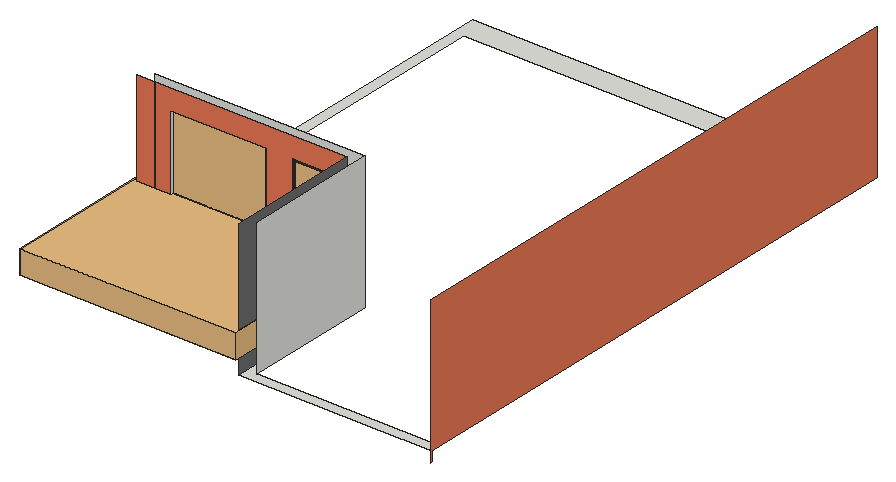
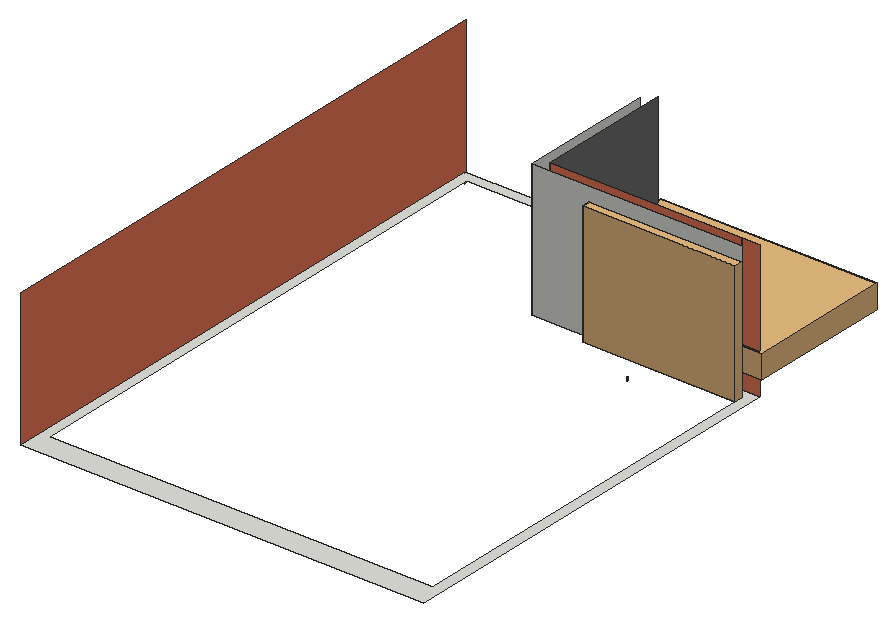
# SketchUp Ruby script. Lengths in inches.
U = 1.inch
M = Sketchup.active_model
def pt(a) = Geom::Point3d.new(a.map { |v| v * U })
def face(e, loops, mat)
  f = e.add_face(loops[0].map { |a| pt(a) })
  loops[1..].each { |l| e.add_face(l.map { |a| pt(a) }).erase! }
  f.material = f.back_material = mat if mat
  f
end
# faces: each face lists its corners as indices into pts; further lists are holes
def faces(e, pts, list, mat = nil) = list.each { |f| face(e, (f[0].is_a?(Array) ? f : [f]).map { |l| l.map { |i| pts[i] } }, mat) }
# xy, xz, yz: faces in a plane at the given z, y or x. An outline is a flat list of corners, or four numbers for a rectangle; further outlines are holes
def ring(l) = l.size == 4 ? [[l[0], l[1]], [l[2], l[1]], [l[2], l[3]], [l[0], l[3]]] : l.each_slice(2).to_a
def flat(e, list, mat, &to3) = list.each { |f| face(e, (f[0].is_a?(Array) ? f : [f]).map { |l| ring(l).map { |u, v| to3.(u, v) } }, mat) }
def xy(e, z, list, mat = nil) = flat(e, list, mat) { |x, y| [x, y, z] }
def xz(e, y, list, mat = nil) = flat(e, list, mat) { |x, z| [x, y, z] }
def yz(e, x, list, mat = nil) = flat(e, list, mat) { |y, z| [x, y, z] }
def lines(e, pts, list) = list.each { |a, b| e.add_line(pt(pts[a]), pt(pts[b])) }
# prism: a flat outline (further loops are holes) pulled along v
def prism(e, loops, v, mat = nil)
  f = face(e, loops, mat); d = Geom::Vector3d.new(v.map { |x| x * U })
  f.pushpull(f.normal.samedirection?(d) ? d.length : -d.length)
end
def box(e, o, s, mat = nil) = prism(e, [[o, [o[0] + s[0], o[1], o[2]], [o[0] + s[0], o[1] + s[1], o[2]], [o[0], o[1] + s[1], o[2]]]], [0, 0, s[2]], mat)
def at(x, y, z, deg = 0) = Geom::Transformation.translation(pt([x, y, z])) * Geom::Transformation.rotation(ORIGIN, Z_AXIS, deg.degrees)
def axes(o, x, y, z) = Geom::Transformation.new([*x, 0, *y, 0, *z, 0, *pt(o).to_a, 1])
def part(name) = M.definitions.add(name)
# library, detail: a bought-in or finely detailed component or shape, given as its bounding box
def library(name, o, s) = part(name).tap { |d| box(d.entities, o, s) }
def detail(e, o, s) = box(e.add_group.entities, o, s)
def put(e, d, t, mat = nil) = e.add_instance(d, t).tap { |i| i.material = mat if mat }
def group(e, t, mat = nil) = e.add_group.tap { |g| g.transformation = t; g.material = mat if mat }.entities
root = M.entities
M.materials.add("1122 AP 7994 PEACH ROSE").color = [254, 227, 201]
M.materials.add("[Formica Beige]").color = [235, 120, 86]
M.materials.add("[Metal Rusted]").color = [135, 86, 63]
M.materials.add("[Stone Flagstone Ashlar]").color = [109, 109, 109]
M.materials.add("[Translucent Glass Blue]1").color = [190, 201, 222]
M.materials["[Translucent Glass Blue]1"].alpha = 0.5
M.materials.add("[Wood Veneer 01]").color = [96, 60, 36]
c1 = library("Group\#47",[0,0,0],[190.94,127,21])
c2 = library("Lattice screen panel",[0,0,-3],[165.74,168.8125,3])
c3 = part("Decorative lattice screen")
put(c3.entities,c2,at(0,0,3))
put(c3.entities,c2,axes([0,675.25,3],[1,0,0],[0,-1,0],[0,0,1]))
put(c3.entities,c2,axes([331.47,0,3],[-1,0,0],[0,1,0],[0,0,1]))
put(c3.entities,c2,at(331.47,675.25,3,180))
put(c3.entities,c2,at(331.47,337.625,3,180))
put(c3.entities,c2,at(0,337.625,3))
put(c3.entities,c2,axes([331.47,337.625,3],[-1,0,0],[0,1,0],[0,0,1]))
put(c3.entities,c2,axes([0,337.625,3],[1,0,0],[0,-1,0],[0,0,1]))
c4 = part("Jali")
put(c4.entities,c3,at(55.22,75.56,-3),"[Metal Rusted]")
g1 = group(c4.entities,at(46.22,66.56,-6))
prism(g1,[[[0,0,0],[0,693.25,0],[349.47,693.25,0],[349.47,0,0]],[[340.47,9,0],[340.47,684.25,0],[9,684.25,0],[9,9,0]]],[0,0,9])
g2 = group(c4.entities,at(46.22,66.56,-15))
g3 = group(g2,at(0,0,0))
prism(g3,[[[0,0,0],[0,693.25,0],[349.47,693.25,0],[349.47,0,0]],[[340.47,9,0],[340.47,684.25,0],[9,684.25,0],[9,9,0]]],[0,0,9])
g4 = group(g2,at(9,9,2.08))
box(g4,[0,0,0],[331.47,675.25,3.9375],"[Translucent Glass Blue]1")
c5 = library("Cửa đi trượt D7",[0,-6.04,0],[84.18,6.04,102])
c6 = library("Component_63",[0,-41.05,1.35],[7.23,156.73,136.43])
xy(root,158.82,[[195,153,195,276,147,276,147,273,123,273,123,282,204,282,204,162,357,162,357,624,18,624,18,282,39,282,39,273,25.25,273,25.25,273.25,25,273.25,25,273,9,273,9,645,366,645,366,153,339.75,153,339.75,153.25,338.75,153.25,338.75,153,321,153,321,153.25,320.75,153.25,320.75,153]])
xz(root,186.05,[[104.56,149.82,104.64,152.82],[105.26,149.82,105.34,152.82],[164.56,149.82,164.64,152.82],[165.26,149.82,165.34,152.82]],"1122 AP 7994 PEACH ROSE")
xz(root,186.07,[[104.79,149.82,104.87,152.82],[104.87,149.82,104.95,152.82],[104.95,149.82,105.03,152.82],[105.03,149.82,105.11,152.82],[164.79,149.82,164.87,152.82],
  [164.87,149.82,164.95,152.82],[164.95,149.82,165.03,152.82],[165.03,149.82,165.11,152.82]],"1122 AP 7994 PEACH ROSE")
xz(root,273,[[9,158.82,25,278.82],[25.25,158.82,39,158.82,39,260.82,123,260.82,123,158.82,147,158.82,147,260.82,195,260.82,195,278.82,25.25,278.82]],"[Formica Beige]")
xz(root,273.25,[[25,158.82,25.25,278.82]])
xz(root,276,[[147,158.82,195,260.82]])
xz(root,282,[[18,158.82,18,278.82,204,278.82,204,158.82,123,158.82,123,260.82,39,260.82,39,158.82]])
xz(root,300.07,[[104.79,149.82,104.87,152.82],[104.87,149.82,104.95,152.82],[104.95,149.82,105.03,152.82],[105.03,149.82,105.11,152.82]],"1122 AP 7994 PEACH ROSE")
yz(root,25,[[273,158.82,273.25,278.82]])
yz(root,25.25,[[273,158.82,273.25,278.82]])
yz(root,39,[[273,158.82,282,260.82]])
yz(root,123,[[273,158.82,282,260.82]])
yz(root,147,[[273,158.82,276,260.82]])
yz(root,195,[[153,158.82,153,278.82,273,278.82,273,260.82,276,260.82,276,158.82]],"[Stone Flagstone Ashlar]")
yz(root,204,[[162,158.82,282,278.82]])
yz(root,366,[[152,149.82,153,149.82,153,158.82,645,158.82,645,278.82,152,278.82,152,243.82,153.25,243.82,153.25,243.57,152,243.57,152,210.82,153.25,210.82,153.25,210.57,152,210.57]],"[Formica Beige]")
p = [[43.65,184.5,149.82],[43.6875,184.43,149.82],[43.6875,184.43,152.82],[43.65,184.5,152.82],[102.28,184.43,149.82],[102.31,184.5,149.82],
  [102.31,184.5,152.82],[102.28,184.43,152.82],[107.59,184.5,149.82],[107.625,184.43,149.82],[107.625,184.43,152.82],[107.59,184.5,152.82],
  [162.24,184.36,149.82],[162.28,184.43,149.82],[162.28,184.43,152.82],[162.24,184.36,152.82],[162.31,184.5,149.82],[162.31,184.5,152.82],
  [167.625,184.43,149.82],[167.66,184.36,149.82],[167.66,184.36,152.82],[167.625,184.43,152.82],[167.59,184.5,149.82],[167.59,184.5,152.82],
  [43.61,184.57,149.82],[43.61,184.57,152.82],[102.35,184.57,149.82],[102.35,184.57,152.82],[107.55,184.57,149.82],[107.55,184.57,152.82],
  [162.35,184.57,149.82],[162.35,184.57,152.82],[167.55,184.57,149.82],[167.55,184.57,152.82],[43.53,184.7,149.82],[43.57,184.64,149.82],
  [43.57,184.64,152.82],[43.53,184.7,152.82],[102.39,184.64,149.82],[102.39,184.64,152.82],[102.44,184.7,149.82],[102.44,184.7,152.82],
  [107.51,184.64,149.82],[107.51,184.64,152.82],[107.47,184.7,149.82],[107.47,184.7,152.82],[162.39,184.64,149.82],[162.39,184.64,152.82],
  [162.44,184.7,149.82],[162.44,184.7,152.82],[167.51,184.64,149.82],[167.51,184.64,152.82],[167.47,184.7,149.82],[167.47,184.7,152.82],
  [43.49,184.77,149.82],[43.49,184.77,152.82],[102.48,184.77,149.82],[102.48,184.77,152.82],[107.42,184.77,149.82],[107.42,184.77,152.82],
  [162.48,184.77,149.82],[162.48,184.77,152.82],[167.42,184.77,149.82],[167.42,184.77,152.82],[43.44,184.83,149.82],[43.44,184.83,152.82],
  [43.4,184.9,149.82],[43.4,184.9,152.82],[102.52,184.83,149.82],[102.52,184.83,152.82],[102.57,184.9,149.82],[102.57,184.9,152.82],
  [107.33,184.9,149.82],[107.38,184.83,149.82],[107.38,184.83,152.82],[107.33,184.9,152.82],[162.52,184.83,149.82],[162.52,184.83,152.82],
  [162.57,184.9,149.82],[162.57,184.9,152.82],[167.33,184.9,149.82],[167.38,184.83,149.82],[167.38,184.83,152.82],[167.33,184.9,152.82],
  [43.35,184.96,149.82],[43.35,184.96,152.82],[102.62,184.96,149.82],[102.62,184.96,152.82],[107.28,184.96,149.82],[107.28,184.96,152.82],
  [162.62,184.96,149.82],[162.62,184.96,152.82],[167.28,184.96,149.82],[167.28,184.96,152.82],[43.25,185.08,149.82],[43.3,185.02,149.82],
  [43.3,185.02,152.82],[43.25,185.08,152.82],[102.67,185.02,149.82],[102.67,185.02,152.82],[102.72,185.08,149.82],[102.72,185.08,152.82],
  [107.23,185.02,149.82],[107.23,185.02,152.82],[107.18,185.08,149.82],[107.18,185.08,152.82],[162.67,185.02,149.82],[162.67,185.02,152.82],
  [162.72,185.08,149.82],[162.72,185.08,152.82],[167.23,185.02,149.82],[167.23,185.02,152.82],[167.18,185.08,149.82],[167.18,185.08,152.82],
  [43.14,185.19,149.82],[43.19,185.14,149.82],[43.19,185.14,152.82],[43.14,185.19,152.82],[102.78,185.14,149.82],[102.78,185.14,152.82],
  [102.83,185.19,149.82],[102.83,185.19,152.82],[107.13,185.14,149.82],[107.13,185.14,152.82],[107.07,185.19,149.82],[107.07,185.19,152.82],
  [162.78,185.14,149.82],[162.78,185.14,152.82],[162.83,185.19,149.82],[162.83,185.19,152.82],[167.13,185.14,149.82],[167.13,185.14,152.82],
  [167.07,185.19,149.82],[167.07,185.19,152.82],[43.02,185.3,149.82],[43.08,185.25,149.82],[43.08,185.25,152.82],[43.02,185.3,152.82],
  [102.89,185.25,149.82],[102.89,185.25,152.82],[102.94,185.3,149.82],[102.94,185.3,152.82],[107.02,185.25,149.82],[107.02,185.25,152.82],
  [106.96,185.3,149.82],[106.96,185.3,152.82],[162.89,185.25,149.82],[162.89,185.25,152.82],[162.94,185.3,149.82],[162.94,185.3,152.82],
  [167.02,185.25,149.82],[167.02,185.25,152.82],[166.96,185.3,149.82],[166.96,185.3,152.82],[42.96,185.35,149.82],[42.96,185.35,152.82],
  [103,185.35,149.82],[103,185.35,152.82],[106.9,185.35,149.82],[106.9,185.35,152.82],[163,185.35,149.82],[163,185.35,152.82],
  [166.9,185.35,149.82],[166.9,185.35,152.82],[42.84,185.45,149.82],[42.9,185.4,149.82],[42.9,185.4,152.82],[42.84,185.45,152.82],
  [103.0625,185.4,149.82],[103.0625,185.4,152.82],[103.125,185.45,149.82],[103.125,185.45,152.82],[106.84,185.4,149.82],[106.84,185.4,152.82],
  [106.78,185.45,149.82],[106.78,185.45,152.82],[163.0625,185.4,149.82],[163.0625,185.4,152.82],[163.125,185.45,149.82],[163.125,185.45,152.82],
  [166.84,185.4,149.82],[166.84,185.4,152.82],[166.78,185.45,149.82],[166.78,185.45,152.82],[42.72,185.54,149.82],[42.78,185.5,149.82],
  [42.78,185.5,152.82],[42.72,185.54,152.82],[42.65,185.59,149.82],[42.65,185.59,152.82],[103.1875,185.5,149.82],[103.1875,185.5,152.82],
  [103.25,185.54,149.82],[103.25,185.54,152.82],[103.32,185.59,149.82],[103.32,185.59,152.82],[106.59,185.59,149.82],[106.65,185.54,149.82],
  [106.65,185.54,152.82],[106.59,185.59,152.82],[106.71,185.5,149.82],[106.71,185.5,152.82],[163.1875,185.5,149.82],[163.1875,185.5,152.82],
  [163.25,185.54,149.82],[163.25,185.54,152.82],[163.32,185.59,149.82],[163.32,185.59,152.82],[166.59,185.59,149.82],[166.65,185.54,149.82],
  [166.65,185.54,152.82],[166.59,185.59,152.82],[166.71,185.5,149.82],[166.71,185.5,152.82],[42.52,185.67,149.82],[42.58,185.63,149.82],
  [42.58,185.63,152.82],[42.52,185.67,152.82],[103.38,185.63,149.82],[103.38,185.63,152.82],[103.45,185.67,149.82],[103.45,185.67,152.82],
  [106.52,185.63,149.82],[106.52,185.63,152.82],[106.45,185.67,149.82],[106.45,185.67,152.82],[163.38,185.63,149.82],[163.38,185.63,152.82],
  [163.45,185.67,149.82],[163.45,185.67,152.82],[166.52,185.63,149.82],[166.52,185.63,152.82],[166.45,185.67,149.82],[166.45,185.67,152.82],
  [42.31,185.78,149.82],[42.38,185.74,149.82],[42.38,185.74,152.82],[42.31,185.78,152.82],[42.45,185.71,149.82],[42.45,185.71,152.82],
  [103.52,185.71,149.82],[103.52,185.71,152.82],[103.59,185.74,149.82],[103.59,185.74,152.82],[103.66,185.78,149.82],[103.66,185.78,152.82],
  [106.24,185.78,149.82],[106.3125,185.74,149.82],[106.3125,185.74,152.82],[106.24,185.78,152.82],[106.38,185.71,149.82],[106.38,185.71,152.82],
  [163.52,185.71,149.82],[163.52,185.71,152.82],[163.59,185.74,149.82],[163.59,185.74,152.82],[163.66,185.78,149.82],[163.66,185.78,152.82],
  [166.24,185.78,149.82],[166.3125,185.74,149.82],[166.3125,185.74,152.82],[166.24,185.78,152.82],[166.38,185.71,149.82],[166.38,185.71,152.82],
  [42.09,185.87,149.82],[42.16,185.84,149.82],[42.16,185.84,152.82],[42.09,185.87,152.82],[42.24,185.8125,149.82],[42.24,185.8125,152.82],
  [103.73,185.8125,149.82],[103.73,185.8125,152.82],[103.8,185.84,149.82],[103.8,185.84,152.82],[103.875,185.87,149.82],[103.875,185.87,152.82],
  [106.03,185.87,149.82],[106.1,185.84,149.82],[106.1,185.84,152.82],[106.03,185.87,152.82],[106.17,185.8125,149.82],[106.17,185.8125,152.82],
  [163.73,185.8125,149.82],[163.73,185.8125,152.82],[163.8,185.84,149.82],[163.8,185.84,152.82],[163.875,185.87,149.82],[163.875,185.87,152.82],
  [166.03,185.87,149.82],[166.1,185.84,149.82],[166.1,185.84,152.82],[166.03,185.87,152.82],[166.17,185.8125,149.82],[166.17,185.8125,152.82],
  [41.79,185.97,149.82],[41.87,185.95,149.82],[41.87,185.95,152.82],[41.79,185.97,152.82],[41.94,185.92,149.82],[42.02,185.9,149.82],
  [42.02,185.9,152.82],[41.94,185.92,152.82],[103.95,185.9,149.82],[103.95,185.9,152.82],[104.02,185.92,149.82],[104.02,185.92,152.82],
  [104.1,185.95,149.82],[104.1,185.95,152.82],[104.17,185.97,149.82],[104.17,185.97,152.82],[105.73,185.97,149.82],[105.8,185.95,149.82],
  [105.8,185.95,152.82],[105.73,185.97,152.82],[105.88,185.92,149.82],[105.88,185.92,152.82],[105.95,185.9,149.82],[105.95,185.9,152.82],
  [163.95,185.9,149.82],[163.95,185.9,152.82],[164.02,185.92,149.82],[164.02,185.92,152.82],[164.1,185.95,149.82],[164.1,185.95,152.82],
  [164.17,185.97,149.82],[164.17,185.97,152.82],[165.73,185.97,149.82],[165.8,185.95,149.82],[165.8,185.95,152.82],[165.73,185.97,152.82],
  [165.88,185.92,149.82],[165.88,185.92,152.82],[165.95,185.9,149.82],[165.95,185.9,152.82],[41.64,186.01,149.82],[41.72,185.99,149.82],
  [41.72,185.99,152.82],[41.64,186.01,152.82],[104.25,185.99,149.82],[104.25,185.99,152.82],[104.33,186.01,149.82],[104.33,186.01,152.82],
  [104.4,186.02,149.82],[104.4,186.02,152.82],[104.48,186.03,149.82],[104.48,186.03,152.82],[104.56,186.05,149.82],[104.56,186.05,152.82],
  [105.34,186.05,149.82],[105.42,186.03,149.82],[105.42,186.03,152.82],[105.34,186.05,152.82],[105.5,186.02,149.82],[105.5,186.02,152.82],
  [105.57,186.01,149.82],[105.57,186.01,152.82],[105.65,185.99,149.82],[105.65,185.99,152.82],[164.25,185.99,149.82],[164.25,185.99,152.82],
  [164.33,186.01,149.82],[164.33,186.01,152.82],[164.4,186.02,149.82],[164.4,186.02,152.82],[164.48,186.03,149.82],[164.48,186.03,152.82],
  [164.56,186.05,149.82],[164.56,186.05,152.82],[165.34,186.05,149.82],[165.42,186.03,149.82],[165.42,186.03,152.82],[165.34,186.05,152.82],
  [165.5,186.02,149.82],[165.5,186.02,152.82],[165.57,186.01,149.82],[165.57,186.01,152.82],[165.65,185.99,149.82],[165.65,185.99,152.82],
  [104.64,186.05,149.82],[104.72,186.0625,149.82],[104.72,186.0625,152.82],[104.64,186.05,152.82],[104.79,186.07,149.82],[104.79,186.07,152.82],
  [105.11,186.07,149.82],[105.1875,186.0625,149.82],[105.1875,186.0625,152.82],[105.11,186.07,152.82],[105.26,186.05,149.82],[105.26,186.05,152.82],
  [164.64,186.05,149.82],[164.72,186.0625,149.82],[164.72,186.0625,152.82],[164.64,186.05,152.82],[164.79,186.07,149.82],[164.79,186.07,152.82],
  [165.11,186.07,149.82],[165.1875,186.0625,149.82],[165.1875,186.0625,152.82],[165.11,186.07,152.82],[165.26,186.05,149.82],[165.26,186.05,152.82],
  [104.56,300.1,149.82],[104.48,300.11,149.82],[104.48,300.11,152.82],[104.56,300.1,152.82],[104.72,300.08,149.82],[104.64,300.09,149.82],
  [104.64,300.09,152.82],[104.72,300.08,152.82],[104.79,300.07,149.82],[104.79,300.07,152.82],[105.1875,300.08,149.82],[105.11,300.07,149.82],
  [105.11,300.07,152.82],[105.1875,300.08,152.82],[105.26,300.09,149.82],[105.26,300.09,152.82],[105.34,300.1,149.82],[105.34,300.1,152.82],
  [105.42,300.11,149.82],[105.42,300.11,152.82],[105.5,300.12,149.82],[105.5,300.12,152.82]]
faces(root,p,[[0,1,2,3],[4,5,6,7],[8,9,10,11],[12,13,14,15],[13,16,17,14],[18,19,20,21],[22,18,21,23],[24,0,3,25],
  [5,26,27,6],[28,8,11,29],[16,30,31,17],[32,22,23,33],[34,35,36,37],[35,24,25,36],[26,38,39,27],[38,40,41,39],
  [42,28,29,43],[44,42,43,45],[30,46,47,31],[46,48,49,47],[50,32,33,51],[52,50,51,53],[54,34,37,55],[40,56,57,41],
  [58,44,45,59],[48,60,61,49],[62,52,53,63],[64,54,55,65],[66,64,65,67],[56,68,69,57],[68,70,71,69],[72,73,74,75],
  [73,58,59,74],[60,76,77,61],[76,78,79,77],[80,81,82,83],[81,62,63,82],[84,66,67,85],[70,86,87,71],[88,72,75,89],
  [78,90,91,79],[92,80,83,93],[94,95,96,97],[95,84,85,96],[86,98,99,87],[98,100,101,99],[102,88,89,103],[104,102,103,105],
  [90,106,107,91],[106,108,109,107],[110,92,93,111],[112,110,111,113],[114,115,116,117],[115,94,97,116],[100,118,119,101],[118,120,121,119],
  [122,104,105,123],[124,122,123,125],[108,126,127,109],[126,128,129,127],[130,112,113,131],[132,130,131,133],[134,135,136,137],[135,114,117,136],
  [120,138,139,121],[138,140,141,139],[142,124,125,143],[144,142,143,145],[128,146,147,129],[146,148,149,147],[150,132,133,151],[152,150,151,153],
  [154,134,137,155],[140,156,157,141],[158,144,145,159],[148,160,161,149],[162,152,153,163],[164,165,166,167],[165,154,155,166],[156,168,169,157],
  [168,170,171,169],[172,158,159,173],[174,172,173,175],[160,176,177,161],[176,178,179,177],[180,162,163,181],[182,180,181,183],[184,185,186,187],
  [188,184,187,189],[185,164,167,186],[170,190,191,171],[190,192,193,191],[192,194,195,193],[196,197,198,199],[200,174,175,201],[197,200,201,198],
  [178,202,203,179],[202,204,205,203],[204,206,207,205],[208,209,210,211],[212,182,183,213],[209,212,213,210],[214,215,216,217],[215,188,189,216],
  [194,218,219,195],[218,220,221,219],[222,196,199,223],[224,222,223,225],[206,226,227,207],[226,228,229,227],[230,208,211,231],[232,230,231,233],
  [234,235,236,237],[238,214,217,239],[235,238,239,236],[220,240,241,221],[240,242,243,241],[242,244,245,243],[246,247,248,249],[247,250,251,248],
  [250,224,225,251],[228,252,253,229],[252,254,255,253],[254,256,257,255],[258,259,260,261],[259,262,263,260],[262,232,233,263],[264,265,266,267],
  [268,234,237,269],[265,268,269,266],[244,270,271,245],[270,272,273,271],[272,274,275,273],[276,277,278,279],[277,280,281,278],[280,246,249,281],
  [256,282,283,257],[282,284,285,283],[284,286,287,285],[288,289,290,291],[289,292,293,290],[292,258,261,293],[294,295,296,297],[298,299,300,301],
  [295,298,301,296],[299,264,267,300],[274,302,303,275],[302,304,305,303],[304,306,307,305],[306,308,309,307],[310,311,312,313],[311,314,315,312],
  [314,316,317,315],[316,276,279,317],[286,318,319,287],[318,320,321,319],[320,322,323,321],[322,324,325,323],[326,327,328,329],[327,330,331,328],
  [330,332,333,331],[332,288,291,333],[334,335,336,337],[335,294,297,336],[308,338,339,309],[338,340,341,339],[340,342,343,341],[342,344,345,343],
  [344,346,347,345],[348,349,350,351],[349,352,353,350],[352,354,355,353],[354,356,357,355],[356,310,313,357],[324,358,359,325],[358,360,361,359],
  [360,362,363,361],[362,364,365,363],[364,366,367,365],[368,369,370,371],[369,372,373,370],[372,374,375,373],[374,376,377,375],[376,326,329,377],
  [378,379,380,381],[379,382,383,380],[384,385,386,387],[385,388,389,386],[390,391,392,393],[391,394,395,392],[396,397,398,399],[397,400,401,398],
  [402,403,404,405],[406,407,408,409],[407,402,405,408],[410,406,409,411],[412,413,414,415],[416,412,415,417],[418,416,417,419],[420,418,419,421],
  [422,420,421,423]],"1122 AP 7994 PEACH ROSE")
put(root,c1,at(6.06,148,173.82))
put(root,c4,axes([140.65,273.86,149.03],[0.13735,0,0],[0,0,0.14713],[0,-0.12,0]),"[Wood Veneer 01]")
put(root,c5,axes([39,275,158.82],[1,0,0],[0,-1,0],[0,0,1]))
put(root,c6,axes([117.64,282,267.67],[0,1,0],[-0.86133,0,0],[0,0,-0.79]))
